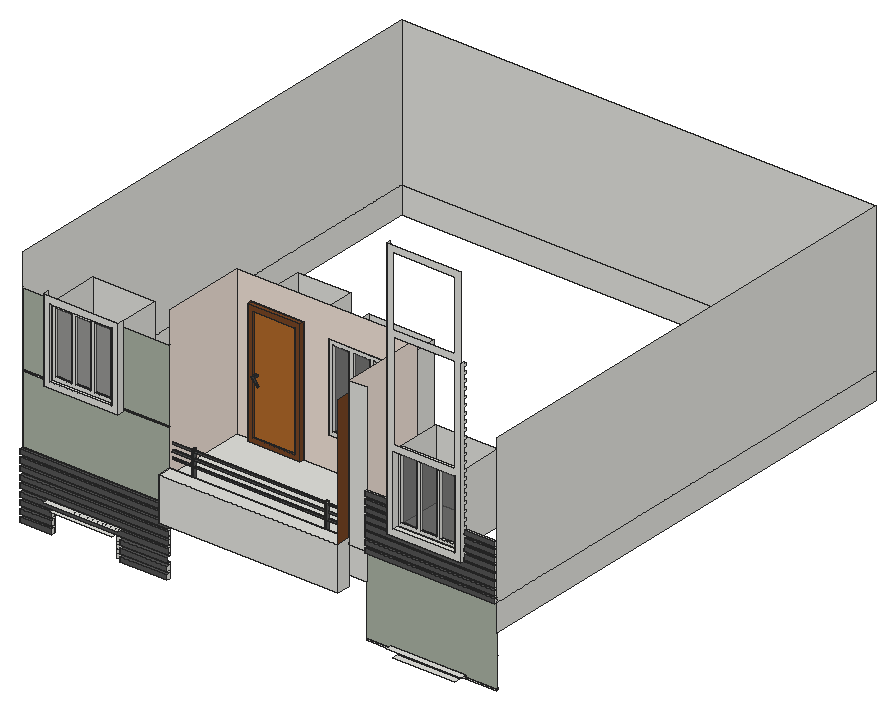
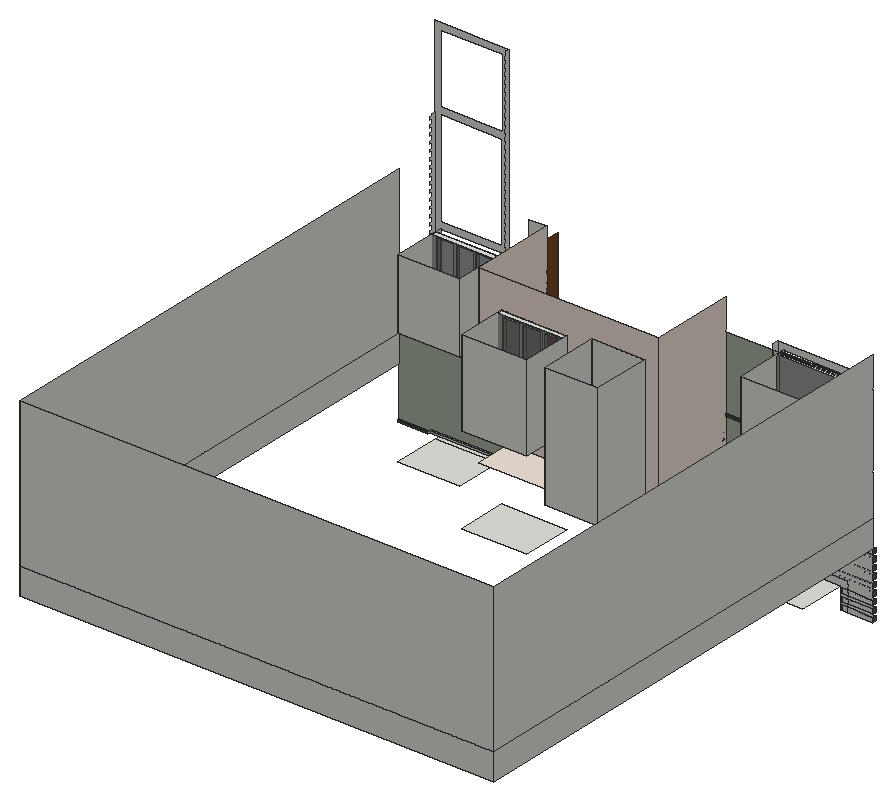
# SketchUp Ruby script. Lengths in inches.
U = 1.inch
M = Sketchup.active_model
def pt(a) = Geom::Point3d.new(a.map { |v| v * U })
def face(e, loops, mat)
  f = e.add_face(loops[0].map { |a| pt(a) })
  loops[1..].each { |l| e.add_face(l.map { |a| pt(a) }).erase! }
  f.material = f.back_material = mat if mat
  f
end
# faces: each face lists its corners as indices into pts; further lists are holes
def faces(e, pts, list, mat = nil) = list.each { |f| face(e, (f[0].is_a?(Array) ? f : [f]).map { |l| l.map { |i| pts[i] } }, mat) }
# xy, xz, yz: faces in a plane at the given z, y or x. An outline is a flat list of corners, or four numbers for a rectangle; further outlines are holes
def ring(l) = l.size == 4 ? [[l[0], l[1]], [l[2], l[1]], [l[2], l[3]], [l[0], l[3]]] : l.each_slice(2).to_a
def flat(e, list, mat, &to3) = list.each { |f| face(e, (f[0].is_a?(Array) ? f : [f]).map { |l| ring(l).map { |u, v| to3.(u, v) } }, mat) }
def xy(e, z, list, mat = nil) = flat(e, list, mat) { |x, y| [x, y, z] }
def xz(e, y, list, mat = nil) = flat(e, list, mat) { |x, z| [x, y, z] }
def yz(e, x, list, mat = nil) = flat(e, list, mat) { |y, z| [x, y, z] }
def lines(e, pts, list) = list.each { |a, b| e.add_line(pt(pts[a]), pt(pts[b])) }
# prism: a flat outline (further loops are holes) pulled along v
def prism(e, loops, v, mat = nil)
  f = face(e, loops, mat); d = Geom::Vector3d.new(v.map { |x| x * U })
  f.pushpull(f.normal.samedirection?(d) ? d.length : -d.length)
end
def box(e, o, s, mat = nil) = prism(e, [[o, [o[0] + s[0], o[1], o[2]], [o[0] + s[0], o[1] + s[1], o[2]], [o[0], o[1] + s[1], o[2]]]], [0, 0, s[2]], mat)
def at(x, y, z, deg = 0) = Geom::Transformation.translation(pt([x, y, z])) * Geom::Transformation.rotation(ORIGIN, Z_AXIS, deg.degrees)
def axes(o, x, y, z) = Geom::Transformation.new([*x, 0, *y, 0, *z, 0, *pt(o).to_a, 1])
def part(name) = M.definitions.add(name)
# library, detail: a bought-in or finely detailed component or shape, given as its bounding box
def library(name, o, s) = part(name).tap { |d| box(d.entities, o, s) }
def detail(e, o, s) = box(e.add_group.entities, o, s)
def put(e, d, t, mat = nil) = e.add_instance(d, t).tap { |i| i.material = mat if mat }
def group(e, t, mat = nil) = e.add_group.tap { |g| g.transformation = t; g.material = mat if mat }.entities
root = M.entities
M.materials.add("Generic\#1").color = [85, 85, 85]
M.materials.add("Generic\#2").color = [170, 178, 163]
M.materials.add("Generic\#4").color = [241, 227, 216]
M.materials.add("[Color M07]").color = [58, 58, 58]
M.materials.add("[Translucent Glass Gray]").color = [91, 91, 91]
M.materials["[Translucent Glass Gray]"].alpha = 0.55
M.materials.add("[Wood Bamboo]").color = [177, 105, 43]
M.materials.add("[Wood Veneer 01]").color = [120, 70, 37]
c1 = part("Group\#4")
xy(c1.entities,0,[[0,0,168,3.625]])
xy(c1.entities,5.375,[[0,0,168,3.625]])
xz(c1.entities,0,[[0,0,168,5.375]])
yz(c1.entities,0,[[0,0,3.625,5.375]])
c2 = part("Group\#3")
xy(c2.entities,0,[[0,4.93,60.125,10.18]])
xy(c2.entities,5.66,[[5.66,4.93,54.46,7.18]],"[Wood Veneer 01]")
xy(c2.entities,68.44,[[8.18,1.47,8.18,7.18,9.93,7.18,9.93,2.62]],"[Color M07]")
xy(c2.entities,70.41,[[8.19,0,9.94,1.15,9.94,7.18,8.19,7.18]],"[Color M07]")
xy(c2.entities,134.78,[[5.66,4.93,54.46,7.18]])
xy(c2.entities,140.4375,[[0,4.93,60.125,10.18]],"[Wood Veneer 01]")
xz(c2.entities,4.93,[[[0,0,60.125,140.4375],[5.66,5.66,54.46,134.78]]],"[Wood Veneer 01]")
xz(c2.entities,7.18,[[[5.66,5.66,54.46,134.78],[8.18,68.44,8.19,70.41,9.94,70.41,9.93,68.44]],[8.18,68.44,8.19,70.41,9.94,70.41,9.93,68.44]],"[Wood Bamboo]")
xz(c2.entities,10.18,[[0,0,60.125,140.4375]])
yz(c2.entities,0,[[4.93,0,10.18,140.4375]],"[Wood Veneer 01]")
yz(c2.entities,5.66,[[4.93,5.66,7.18,134.78]],"[Wood Veneer 01]")
yz(c2.entities,54.46,[[4.93,5.66,7.18,134.78]],"[Wood Veneer 01]")
yz(c2.entities,60.125,[[4.93,0,10.18,140.4375]],"[Wood Veneer 01]")
p = [[8.19,0,70.41],[8.18,1.47,68.44],[14.45,1.47,61.21],[15.43,0,62.06],[15.45,2.62,62.07],[16.43,1.15,62.92],
  [9.93,2.62,68.44],[9.94,1.15,70.41],[8.19,7.18,70.41],[8.18,7.18,68.44],[9.93,7.18,68.44],[9.94,7.18,70.41],
  [8.95,0.93,69.83],[15.58,0.93,62.1875],[8.95,7.18,69.83]]
faces(c2.entities,p,[[0,1,2,3],[3,2,4,5],[1,6,4,2],[7,0,3,5],[6,7,5,4],[8,9,1,0],[10,11,7,6]],"[Color M07]")
lines(c2.entities,p,[[12,13],[14,12]])
c3 = part("Group\#2")
xy(c3.entities,0,[[0,0,74.5625,5.5]])
xy(c3.entities,4.83,[[4.83,0,23.24,2.5],[28.07,0,46.49,2.5],[51.32,0,69.73,2.5]])
xy(c3.entities,93.17,[[4.83,0,23.24,2.5],[28.07,0,46.49,2.5],[51.32,0,69.73,2.5]])
xy(c3.entities,98,[[0,0,74.5625,5.5]])
xz(c3.entities,0,[[[0,0,74.5625,98],[28.07,4.83,46.49,93.17],[51.32,4.83,69.73,93.17],[4.83,4.83,23.24,93.17]]])
xz(c3.entities,2.5,[[4.83,4.83,23.24,93.17],[28.07,4.83,46.49,93.17],[51.32,4.83,69.73,93.17]],"[Translucent Glass Gray]")
xz(c3.entities,5.5,[[0,0,74.5625,98]],"[Translucent Glass Gray]")
yz(c3.entities,0,[[0,0,5.5,98]])
yz(c3.entities,4.83,[[0,4.83,2.5,93.17]])
yz(c3.entities,23.24,[[0,4.83,2.5,93.17]])
yz(c3.entities,28.07,[[0,4.83,2.5,93.17]])
yz(c3.entities,46.49,[[0,4.83,2.5,93.17]])
yz(c3.entities,51.32,[[0,4.83,2.5,93.17]])
yz(c3.entities,69.73,[[0,4.83,2.5,93.17]])
yz(c3.entities,74.5625,[[0,0,5.5,98]])
c4 = part("Group\#1")
xy(c4.entities,0,[[0,0,70.8125,6.0625]])
xy(c4.entities,4.26,[[4.26,0,22.19,2.0625],[26.44,0,44.37,2.0625],[48.63,0,66.56,2.0625]])
xy(c4.entities,75.06,[[4.26,0,22.19,2.0625],[26.44,0,44.37,2.0625],[48.63,0,66.56,2.0625]])
xy(c4.entities,79.3125,[[0,0,70.8125,6.0625]])
xz(c4.entities,0,[[[0,0,70.8125,79.3125],[26.44,4.26,44.37,75.06],[4.26,4.26,22.19,75.06],[48.63,4.26,66.56,75.06]]])
xz(c4.entities,2.0625,[[4.26,4.26,22.19,75.06],[26.44,4.26,44.37,75.06],[48.63,4.26,66.56,75.06]],"[Translucent Glass Gray]")
xz(c4.entities,6.0625,[[0,0,70.8125,79.3125]],"[Translucent Glass Gray]")
yz(c4.entities,0,[[0,0,6.0625,79.3125]])
yz(c4.entities,4.26,[[0,4.26,2.0625,75.06]])
yz(c4.entities,22.19,[[0,4.26,2.0625,75.06]])
yz(c4.entities,26.44,[[0,4.26,2.0625,75.06]])
yz(c4.entities,44.37,[[0,4.26,2.0625,75.06]])
yz(c4.entities,48.63,[[0,4.26,2.0625,75.06]])
yz(c4.entities,66.56,[[0,4.26,2.0625,75.06]])
yz(c4.entities,70.8125,[[0,0,6.0625,79.3125]])
xy(root,490.875,[[118.35,26.9375,171.6875,31.0625],[3.6875,27.4375,39.68,31.0625]],"Generic\#1")
xy(root,496.25,[[118.35,26.9375,171.6875,31.0625],[3.6875,27.4375,39.68,31.0625]],"Generic\#1")
xy(root,499.5625,[[118.35,27,171.6875,31.0625],[3.6875,27.4375,39.68,31.0625]],"Generic\#1")
xy(root,503.95,[[430.99,24.0625,501.8,31.0625],[430.99,31.0625,501.8,85.4375]])
xy(root,504.9375,[[118.35,27,171.6875,31.0625],[3.6875,27.4375,39.68,31.0625]],"Generic\#1")
xy(root,507.02,[[395.4375,31.0625,423.8125,32.9375],[508.98,31.0625,543.6875,32.9375]])
xy(root,508.25,[[118.35,27,171.6875,27.4375]])
xy(root,508.25,[[3.6875,27.4375,39.68,31.0625],[118.35,27.4375,171.6875,31.0625]],"Generic\#1")
xy(root,509.02,[[395.4375,31.0625,423.8125,32.9375],[508.98,31.0625,543.6875,32.9375]])
xy(root,511.13,[[423.8125,24.0625,508.98,31.0625]])
xy(root,513.625,[[118.35,27,171.6875,31.0625],[3.6875,27.4375,39.68,31.0625]],"Generic\#1")
xy(root,515.52,[[40.36,24.0625,111.18,31.0625],[40.36,31.0625,111.18,85.4375]])
xy(root,522.69,[[33.1875,24.0625,118.35,31.0625]])
xy(root,532.04,[[275.98,127,350.54,183.625]])
xy(root,538.1875,[[187.38,127,247.51,193.75]])
xy(root,554.25,[[171.6875,15.8125,375.6875,31.0625]])
xy(root,565.75,[[171.6875,31.0625,375.6875,127]],"Generic\#4")
xy(root,596.625,[[[171.6875,31.0625,171.6875,127,187.38,127,187.38,193.75,247.51,193.75,247.51,127,375.6875,127,375.6875,31.0625],[194.79,33.15,196.93,36.37],[346.67,33.15,348.8,36.37]],[194.79,33.15,196.93,36.37],[346.67,33.15,348.8,36.37]])
xy(root,596.625,[[395.4375,28.5,543.6875,31.0625]],"Generic\#1")
xy(root,602.125,[[395.4375,28.5,543.6875,31.0625]],"Generic\#1")
xy(root,603.625,[[171.6875,15.8125,375.6875,31.0625]])
xy(root,604.9375,[[395.4375,28.5,543.6875,31.0625]],"Generic\#1")
xy(root,610.4375,[[395.4375,28.5,543.6875,31.0625]],"Generic\#1")
xy(root,611.4375,[[171.6875,33.8125,375.6875,35.625]],"Generic\#1")
xy(root,613.0625,[[171.6875,33.8125,375.6875,35.625]],"Generic\#1")
xy(root,613.25,[[395.4375,28.5,543.6875,31.0625]],"Generic\#1")
xy(root,618.75,[[395.4375,28.5,543.6875,31.0625]],"Generic\#1")
xy(root,619.1875,[[171.6875,33.8125,375.6875,35.625]],"Generic\#1")
xy(root,620.8125,[[171.6875,33.8125,375.6875,35.625]],"Generic\#1")
xy(root,621.5625,[[395.4375,28.5,543.6875,31.0625]],"Generic\#1")
xy(root,627.0625,[[395.4375,28.5,543.6875,31.0625],[171.6875,33.8125,375.6875,35.625]],"Generic\#1")
xy(root,628.53,[[423.8125,24.0625,508.98,31.0625]])
xy(root,628.6875,[[194.79,33.8125,196.93,35.625],[194.79,35.625,196.93,36.37],[346.67,35.625,348.8,36.37]])
xy(root,628.6875,[[171.6875,33.8125,194.79,35.625],[196.93,33.8125,346.67,35.625],[348.8,33.8125,375.6875,35.625]],"Generic\#1")
xy(root,629.875,[[395.4375,28.5,423.8125,31.0625],[508.98,28.5,543.6875,31.0625]],"Generic\#1")
xy(root,630.1875,[[194.79,33.15,196.93,36.37],[346.67,33.15,348.8,36.37]],"Generic\#1")
xy(root,632.04,[[275.98,127,350.54,183.625]])
xy(root,635.375,[[395.4375,28.5,423.8125,31.0625],[508.98,28.5,543.6875,31.0625]],"Generic\#1")
xy(root,635.7,[[430.99,24.0625,501.8,31.0625],[430.99,31.0625,501.8,85.4375]])
xy(root,638.1875,[[395.4375,28.5,423.8125,31.0625],[508.98,28.5,543.6875,31.0625]],"Generic\#1")
xy(root,641.71,[[33.1875,24.0625,118.35,31.0625]])
xy(root,643.6875,[[395.4375,28.5,423.8125,31.0625],[508.98,28.5,543.6875,31.0625]],"Generic\#1")
xy(root,644.15,[[3.6875,31.0625,33.1875,32.9375],[118.35,31.0625,154.5,32.9375],[154.5,31.0625,171.6875,32.9375]])
xy(root,646.15,[[3.6875,31.0625,33.1875,32.9375],[118.35,31.0625,154.5,32.9375],[154.5,31.0625,171.6875,32.9375]])
xy(root,646.5,[[395.4375,28.5,423.8125,31.0625],[508.98,28.5,543.6875,31.0625]],"Generic\#1")
xy(root,648.89,[[40.36,24.0625,111.18,31.0625],[40.36,31.0625,111.18,85.4375]])
xy(root,652,[[395.4375,28.5,423.8125,31.0625],[508.98,28.5,543.6875,31.0625]],"Generic\#1")
xy(root,654.8125,[[395.4375,28.5,423.8125,31.0625],[508.98,28.5,543.6875,31.0625]],"Generic\#1")
xz(root,15.8125,[[171.6875,554.25,375.6875,603.625]])
xz(root,24.0625,[[[423.8125,628.53,508.98,925.19],[431.91,722.19,501.98,831.53],[430.99,635.7,501.8,715.02],[430.99,838.7,501.8,918.02]],[[33.1875,641.71,118.35,735.38],[40.36,648.89,111.18,728.2]]])
xz(root,26.9375,[[118.35,490.875,171.6875,496.25]],"Generic\#1")
xz(root,27,[[118.35,499.5625,171.6875,504.9375],[118.35,508.25,171.6875,513.625]],"Generic\#1")
xz(root,27.4375,[[3.6875,490.875,39.68,496.25],[3.6875,499.5625,39.68,504.9375],[3.6875,508.25,39.68,513.625]],"Generic\#1")
xz(root,28.5,[[395.4375,596.625,543.6875,602.125],[395.4375,604.9375,543.6875,610.4375],[395.4375,613.25,543.6875,618.75],[395.4375,621.5625,543.6875,627.0625],[395.4375,629.875,423.8125,635.375],
  [508.98,629.875,543.6875,635.375],[395.4375,638.1875,423.8125,643.6875],[508.98,638.1875,543.6875,643.6875],[395.4375,646.5,423.8125,652],[508.98,646.5,543.6875,652],
  [395.4375,654.8125,423.8125,660.3125],[508.98,654.8125,543.6875,660.3125]],"Generic\#1")
xz(root,31.0625,[[3.6875,490.875,33.1875,496.25],[33.1875,490.875,39.68,496.25],[39.68,490.875,40.36,496.25],[111.18,490.875,118.35,496.25],[118.35,490.875,171.6875,496.25],
  [3.6875,496.25,33.1875,499.5625],[33.1875,496.25,40.36,499.5625],[111.18,496.25,118.35,499.5625],[118.35,496.25,171.6875,499.5625],[3.6875,499.5625,33.1875,504.9375],
  [33.1875,499.5625,39.68,504.9375],[39.68,499.5625,40.36,504.9375],[111.18,499.5625,118.35,504.9375],[118.35,499.5625,171.6875,504.9375],[3.6875,504.9375,33.1875,508.25],
  [33.1875,504.9375,40.36,508.25],[111.18,504.9375,118.35,508.25],[118.35,504.9375,171.6875,508.25],[423.8125,507.02,508.98,509.02],[3.6875,508.25,33.1875,513.625],
  [33.1875,508.25,39.68,513.625],[39.68,508.25,40.36,513.625],[111.18,508.25,118.35,513.625],[423.8125,509.02,508.98,511.13],[3.6875,513.625,33.1875,513.625,33.1875,522.69,118.35,522.69,118.35,513.625,171.6875,513.625,171.6875,560.375,3.6875,560.375],
  [33.1875,513.625,33.1875,522.69,118.35,522.69,118.35,513.625,111.18,513.625,111.18,515.52,40.36,515.52,40.36,513.625],[171.6875,554.25,375.6875,565.75],[3.6875,560.375,171.6875,565.75],[171.6875,565.75,375.6875,596.625],[375.6875,565.75,395.4375,596.625],
  [171.6875,596.625,375.6875,603.625],[375.6875,596.625,395.4375,764.625],[395.4375,596.625,543.6875,602.125],[395.4375,602.125,543.6875,604.9375],[395.4375,604.9375,543.6875,610.4375],
  [395.4375,610.4375,543.6875,613.25],[395.4375,613.25,543.6875,618.75],[395.4375,618.75,543.6875,621.5625],[395.4375,621.5625,543.6875,627.0625],[395.4375,627.0625,543.6875,627.0625,543.6875,629.875,508.98,629.875,508.98,628.53,423.8125,628.53,423.8125,629.875,395.4375,629.875],
  [423.8125,628.53,508.98,629.875],[395.4375,629.875,423.8125,635.375],[423.8125,629.875,508.98,635.375],[508.98,629.875,543.6875,635.375],[395.4375,635.375,423.8125,638.1875],
  [423.8125,635.375,423.8125,638.1875,430.99,638.1875,430.99,635.7,501.8,635.7,501.8,638.1875,508.98,638.1875,508.98,635.375],[508.98,635.375,543.6875,638.1875],[395.4375,638.1875,423.8125,643.6875],[423.8125,638.1875,430.99,643.6875],[501.8,638.1875,508.98,643.6875],
  [508.98,638.1875,543.6875,643.6875],[33.1875,641.71,118.35,644.15],[395.4375,643.6875,423.8125,646.5],[423.8125,643.6875,430.99,646.5],[501.8,643.6875,508.98,646.5],
  [508.98,643.6875,543.6875,646.5],[33.1875,644.15,118.35,646.15],[33.1875,646.15,118.35,728.625],[395.4375,646.5,423.8125,652],[423.8125,646.5,430.99,652],
  [501.8,646.5,508.98,652],[508.98,646.5,543.6875,652],[395.4375,652,423.8125,654.8125],[423.8125,652,430.99,654.8125],[501.8,652,508.98,654.8125],
  [508.98,652,543.6875,654.8125],[395.4375,654.8125,423.8125,660.3125],[423.8125,654.8125,430.99,660.3125],[501.8,654.8125,508.98,660.3125],[508.98,654.8125,543.6875,660.3125]])
xz(root,31.0625,[[395.4375,509.02,423.8125,509.02,423.8125,511.13,508.98,511.13,508.98,509.02,543.6875,509.02,543.6875,596.625,395.4375,596.625],[3.6875,565.75,171.6875,565.75,171.6875,644.15,118.35,644.15,118.35,641.71,33.1875,641.71,33.1875,644.15,3.6875,644.15],[33.1875,644.15,33.1875,728.625,3.6875,728.625,3.6875,646.15,171.6875,646.15,171.6875,728.625,118.35,728.625,118.35,644.15]],"Generic\#2")
xz(root,32.9375,[[395.4375,507.02,423.8125,509.02],[508.98,507.02,543.6875,509.02],[3.6875,644.15,33.1875,646.15],[118.35,644.15,171.6875,646.15]],"Generic\#1")
xz(root,33.15,[[194.79,596.625,196.93,630.1875],[346.67,596.625,348.8,630.1875]],"Generic\#1")
xz(root,33.8125,[[171.6875,611.4375,375.6875,613.0625],[171.6875,619.1875,375.6875,620.8125],[171.6875,627.0625,375.6875,628.6875]],"Generic\#1")
xz(root,35.625,[[171.6875,611.4375,375.6875,613.0625],[171.6875,619.1875,375.6875,620.8125],[171.6875,627.0625,375.6875,628.6875]])
xz(root,36.37,[[194.79,596.625,196.93,628.6875],[346.67,596.625,348.8,628.6875],[194.79,628.6875,196.93,630.1875],[346.67,628.6875,348.8,630.1875]])
xz(root,85.4375,[[430.99,635.7,501.8,715.02],[40.36,648.89,111.18,728.2]])
xz(root,127,[[[171.6875,596.625,187.38,596.625,187.38,737.0625,247.51,737.0625,247.51,596.625,375.6875,596.625,375.6875,764.625,171.6875,764.625],[275.98,632.04,350.54,730.04]]],"Generic\#4")
xz(root,183.625,[[275.98,632.04,350.54,730.04]])
xz(root,193.75,[[187.38,596.625,247.51,737.0625]])
xz(root,571.0625,[[3.6875,565.75,543.6875,596.625],[3.6875,596.625,543.6875,764.625]])
yz(root,3.6875,[[31.0625,565.75,571.0625,596.625],[31.0625,596.625,31.0625,644.15,32.9375,644.15,32.9375,646.15,31.0625,646.15,31.0625,728.625,32.9375,728.625,32.9375,730.625,31.0625,730.625,31.0625,764.625,571.0625,764.625,571.0625,596.625]])
yz(root,3.6875,[[27.4375,490.875,31.0625,496.25],[27.4375,499.5625,31.0625,504.9375],[27.4375,508.25,31.0625,513.625]],"Generic\#1")
yz(root,33.1875,[[24.0625,641.71,31.0625,735.38],[31.0625,644.15,32.9375,646.15]])
yz(root,39.68,[[27.4375,490.875,31.0625,496.25],[27.4375,499.5625,31.0625,504.9375],[27.4375,508.25,31.0625,513.625]])
yz(root,40.36,[[24.0625,648.89,31.0625,728.2],[31.0625,648.89,85.4375,728.2]])
yz(root,111.18,[[24.0625,648.89,31.0625,728.2],[31.0625,648.89,85.4375,728.2]])
yz(root,118.35,[[26.9375,490.875,31.0625,496.25],[27,499.5625,31.0625,504.9375],[27,508.25,27.4375,513.625],[27.4375,508.25,31.0625,513.625],[24.0625,641.71,31.0625,735.38],
  [31.0625,644.15,32.9375,646.15]])
yz(root,171.6875,[[26.9375,490.875,31.0625,496.25],[27,499.5625,31.0625,504.9375],[15.8125,554.25,15.8125,603.625,31.0625,603.625,31.0625,565.75,27.4375,565.75,27.4375,560.375,31.0625,560.375,31.0625,554.25],[27.4375,560.375,31.0625,565.75],[33.8125,611.4375,35.625,613.0625],
  [33.8125,619.1875,35.625,620.8125],[33.8125,627.0625,35.625,628.6875]])
yz(root,171.6875,[[[31.0625,596.625,127,596.625,127,764.625,31.0625,764.625,31.0625,730.625,32.9375,730.625,32.9375,728.625,31.0625,728.625,31.0625,646.15,32.9375,646.15,32.9375,644.15,31.0625,644.15],[33.8125,611.4375,35.625,613.0625],[33.8125,619.1875,35.625,620.8125],[33.8125,627.0625,35.625,628.6875]]],"Generic\#4")
yz(root,187.38,[[127,596.625,193.75,737.0625]])
yz(root,194.79,[[33.15,596.625,36.37,628.6875],[33.15,628.6875,33.8125,630.1875],[33.8125,628.6875,35.625,630.1875],[35.625,628.6875,36.37,630.1875]],"Generic\#1")
yz(root,196.93,[[33.15,596.625,36.37,628.6875],[33.15,628.6875,33.8125,630.1875],[33.8125,628.6875,35.625,630.1875],[35.625,628.6875,36.37,630.1875]],"Generic\#1")
yz(root,247.51,[[127,596.625,193.75,737.0625]])
yz(root,275.98,[[127,632.04,183.625,730.04]])
yz(root,346.67,[[33.15,596.625,33.15,630.1875,33.8125,630.1875,33.8125,628.6875,36.37,628.6875,36.37,596.625],[33.8125,628.6875,35.625,630.1875],[35.625,628.6875,36.37,630.1875]],"Generic\#1")
yz(root,348.8,[[33.15,628.6875,33.8125,630.1875],[33.8125,628.6875,35.625,630.1875],[35.625,628.6875,36.37,630.1875]])
yz(root,348.8,[[33.15,596.625,36.37,628.6875]],"Generic\#1")
yz(root,350.54,[[127,632.04,183.625,730.04]])
yz(root,375.6875,[[15.8125,554.25,31.0625,603.625]])
yz(root,375.6875,[[[31.0625,596.625,127,764.625],[33.8125,611.4375,35.625,613.0625],[33.8125,619.1875,35.625,620.8125],[33.8125,627.0625,35.625,628.6875]]],"Generic\#4")
yz(root,375.6875,[[15.8125,603.625,31.0625,751.4375]],"[Wood Veneer 01]")
yz(root,395.4375,[[31.0625,507.02,32.9375,509.02],[28.5,596.625,31.0625,602.125],[28.5,604.9375,31.0625,610.4375],[28.5,613.25,31.0625,618.75],[28.5,621.5625,31.0625,627.0625],
  [28.5,629.875,31.0625,635.375],[28.5,638.1875,31.0625,643.6875],[28.5,646.5,31.0625,652],[28.5,654.8125,31.0625,660.3125]])
yz(root,423.8125,[[31.0625,507.02,32.9375,509.02],[24.0625,628.53,24.0625,925.19,28.5,925.19,28.5,920.8125,31.0625,920.8125,31.0625,918,28.5,918,28.5,912.5,31.0625,912.5,31.0625,909.6875,28.5,909.6875,28.5,904.1875,31.0625,904.1875,31.0625,901.375,28.5,901.375,28.5,895.875,31.0625,895.875,31.0625,893.0625,28.5,893.0625,28.5,887.5625,31.0625,887.5625,31.0625,884.75,28.5,884.75,28.5,879.25,31.0625,879.25,31.0625,876.4375,28.5,876.4375,28.5,870.9375,31.0625,870.9375,31.0625,868.125,28.5,868.125,28.5,862.625,31.0625,862.625,31.0625,859.8125,28.5,859.8125,28.5,854.3125,31.0625,854.3125,31.0625,851.5,28.5,851.5,28.5,846,31.0625,846,31.0625,843.1875,28.5,843.1875,28.5,837.6875,31.0625,837.6875,31.0625,834.875,28.5,834.875,28.5,829.375,31.0625,829.375,31.0625,826.5625,28.5,826.5625,28.5,821.0625,31.0625,821.0625,31.0625,818.25,28.5,818.25,28.5,812.75,31.0625,812.75,31.0625,809.9375,28.5,809.9375,28.5,804.4375,31.0625,804.4375,31.0625,801.625,28.5,801.625,28.5,796.125,31.0625,796.125,31.0625,793.3125,28.5,793.3125,28.5,787.8125,31.0625,787.8125,31.0625,785,28.5,785,28.5,779.5,31.0625,779.5,31.0625,776.6875,28.5,776.6875,28.5,771.1875,31.0625,771.1875,31.0625,768.375,28.5,768.375,28.5,762.875,31.0625,762.875,31.0625,760.0625,28.5,760.0625,28.5,754.5625,31.0625,754.5625,31.0625,751.75,28.5,751.75,28.5,746.25,31.0625,746.25,31.0625,743.4375,28.5,743.4375,28.5,737.9375,31.0625,737.9375,31.0625,735.125,28.5,735.125,28.5,729.625,31.0625,729.625,31.0625,726.8125,28.5,726.8125,28.5,721.3125,31.0625,721.3125,31.0625,718.5,28.5,718.5,28.5,713,31.0625,713,31.0625,710.1875,28.5,710.1875,28.5,704.6875,31.0625,704.6875,31.0625,701.875,28.5,701.875,28.5,696.375,31.0625,696.375,31.0625,693.5625,28.5,693.5625,28.5,688.0625,31.0625,688.0625,31.0625,685.25,28.5,685.25,28.5,679.75,31.0625,679.75,31.0625,676.9375,28.5,676.9375,28.5,671.4375,31.0625,671.4375,31.0625,668.625,28.5,668.625,28.5,663.125,31.0625,663.125,31.0625,660.3125,28.5,660.3125,28.5,654.8125,31.0625,654.8125,31.0625,652,28.5,652,28.5,646.5,31.0625,646.5,31.0625,643.6875,28.5,643.6875,28.5,638.1875,31.0625,638.1875,31.0625,635.375,28.5,635.375,28.5,629.875,31.0625,629.875,31.0625,628.53],[28.5,629.875,31.0625,635.375],[28.5,638.1875,31.0625,643.6875],[28.5,646.5,31.0625,652],
  [28.5,654.8125,31.0625,660.3125]])
yz(root,430.99,[[24.0625,635.7,31.0625,715.02],[31.0625,635.7,85.4375,715.02]])
yz(root,501.8,[[24.0625,635.7,31.0625,715.02],[31.0625,635.7,85.4375,715.02]])
yz(root,508.98,[[31.0625,507.02,32.9375,509.02],[24.0625,628.53,31.0625,628.53,31.0625,629.875,28.5,629.875,28.5,635.375,31.0625,635.375,31.0625,638.1875,28.5,638.1875,28.5,643.6875,31.0625,643.6875,31.0625,646.5,28.5,646.5,28.5,652,31.0625,652,31.0625,654.8125,28.5,654.8125,28.5,660.3125,31.0625,660.3125,31.0625,663.125,28.5,663.125,28.5,668.625,31.0625,668.625,31.0625,671.4375,28.5,671.4375,28.5,676.9375,31.0625,676.9375,31.0625,679.75,28.5,679.75,28.5,685.25,31.0625,685.25,31.0625,688.0625,28.5,688.0625,28.5,693.5625,31.0625,693.5625,31.0625,696.375,28.5,696.375,28.5,701.875,31.0625,701.875,31.0625,704.6875,28.5,704.6875,28.5,710.1875,31.0625,710.1875,31.0625,713,28.5,713,28.5,718.5,31.0625,718.5,31.0625,721.3125,28.5,721.3125,28.5,726.8125,31.0625,726.8125,31.0625,729.625,28.5,729.625,28.5,735.125,31.0625,735.125,31.0625,737.9375,28.5,737.9375,28.5,743.4375,31.0625,743.4375,31.0625,746.25,28.5,746.25,28.5,751.75,31.0625,751.75,31.0625,754.5625,28.5,754.5625,28.5,760.0625,31.0625,760.0625,31.0625,762.875,28.5,762.875,28.5,768.375,31.0625,768.375,31.0625,771.1875,28.5,771.1875,28.5,776.6875,31.0625,776.6875,31.0625,779.5,28.5,779.5,28.5,785,31.0625,785,31.0625,787.8125,28.5,787.8125,28.5,793.3125,31.0625,793.3125,31.0625,796.125,28.5,796.125,28.5,801.625,31.0625,801.625,31.0625,804.4375,28.5,804.4375,28.5,809.9375,31.0625,809.9375,31.0625,812.75,28.5,812.75,28.5,818.25,31.0625,818.25,31.0625,821.0625,28.5,821.0625,28.5,826.5625,31.0625,826.5625,31.0625,829.375,28.5,829.375,28.5,831.53,24.0625,831.53],[28.5,629.875,31.0625,635.375],[28.5,638.1875,31.0625,643.6875],[28.5,646.5,31.0625,652],
  [28.5,654.8125,31.0625,660.3125]])
yz(root,543.6875,[[31.0625,565.75,571.0625,596.625],[28.5,596.625,31.0625,602.125],[31.0625,596.625,571.0625,764.625],[28.5,604.9375,31.0625,610.4375],[28.5,613.25,31.0625,618.75],
  [28.5,621.5625,31.0625,627.0625],[28.5,629.875,31.0625,635.375],[28.5,638.1875,31.0625,643.6875],[28.5,646.5,31.0625,652],[28.5,654.8125,31.0625,660.3125]])
p = [[171.6875,34.74,612.24],[195.84,34.74,612.24],[171.6875,34.74,620.11],[195.84,34.74,620.11],[171.6875,34.74,627.99],[195.84,34.74,627.99],
  [347.53,34.74,627.99],[375.6875,34.74,627.99],[347.53,34.74,620.11],[347.53,34.74,612.24],[375.6875,34.74,612.24],[375.6875,34.74,620.11],
  [347.53,34.74,603.625],[195.84,34.74,603.625],[195.84,34.74,596.625],[347.53,34.74,596.625],[39.68,27.4375,513.625],[40.36,27.4375,513.625],
  [39.68,27.4375,499.5625],[40.36,27.4375,499.5625],[39.68,27.4375,490.875],[40.36,27.4375,490.875]]
lines(root,p,[[0,1],[2,3],[4,5],[6,7],[6,8],[9,10],[8,11],[9,12],[8,9],[5,3],[1,13],[3,1],
  [1,9],[3,8],[5,6],[13,14],[12,15],[16,17],[18,19],[20,21]])
put(root,c1,at(3.6875,27.4375,516.9375),"Generic\#1")
put(root,c1,at(3.6875,27.4375,525.625),"Generic\#1")
put(root,c1,at(3.6875,27.4375,534.3125),"Generic\#1")
put(root,c1,at(3.6875,27.4375,543),"Generic\#1")
put(root,c1,at(3.6875,27.4375,551.6875),"Generic\#1")
put(root,c1,at(3.6875,27.4375,560.375),"Generic\#1")
put(root,c2,at(187.38,116.82,596.625))
put(root,c3,at(275.98,127,632.04))
put(root,c4,at(430.99,31.0625,635.7))
put(root,c4,at(40.36,27.5625,648.89))
